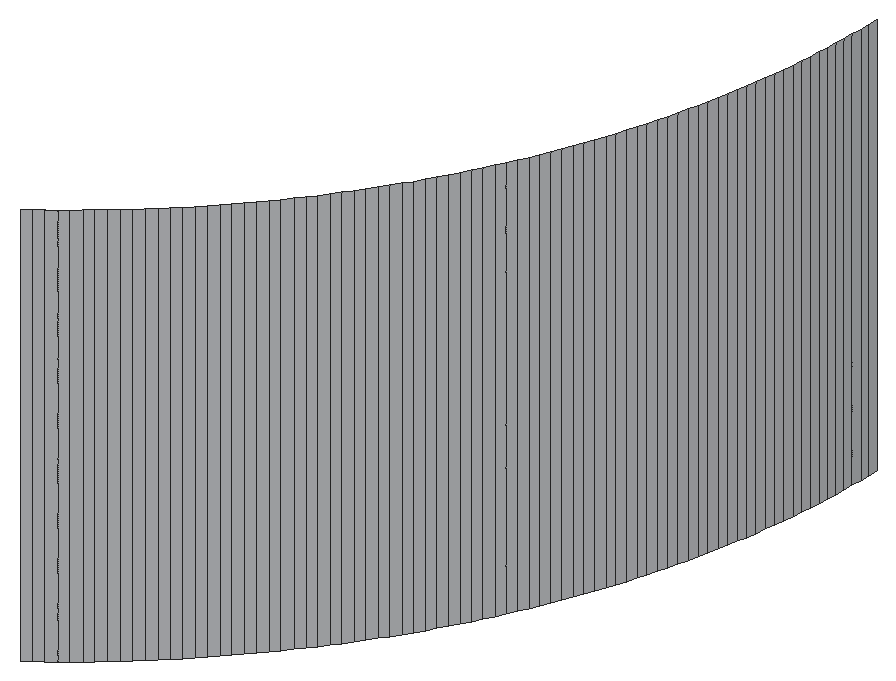
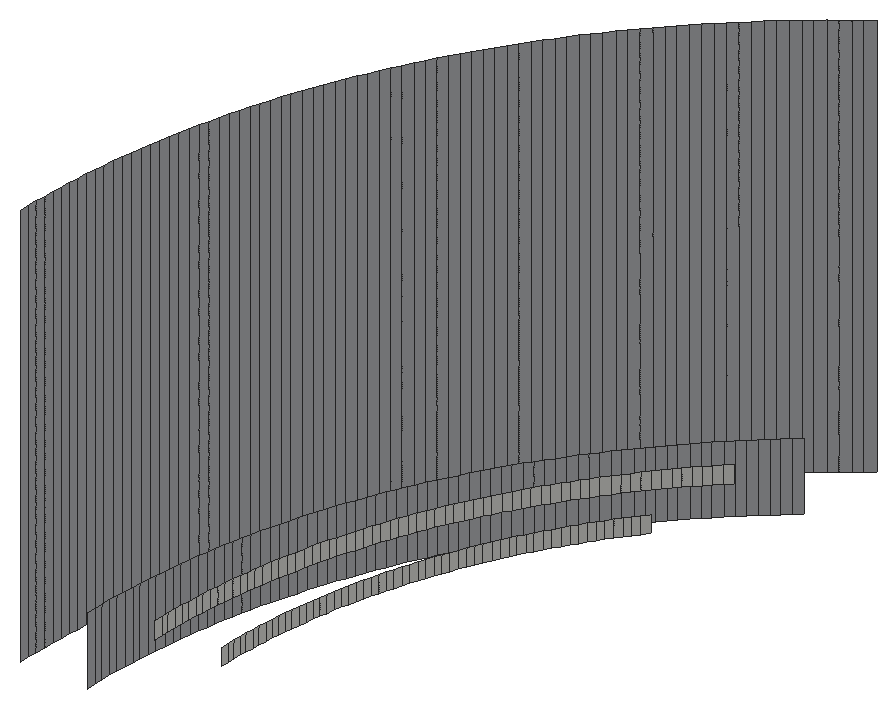
# SketchUp Ruby script. Lengths in inches.
U = 1.inch
M = Sketchup.active_model
def pt(a) = Geom::Point3d.new(a.map { |v| v * U })
def face(e, loops, mat)
  f = e.add_face(loops[0].map { |a| pt(a) })
  loops[1..].each { |l| e.add_face(l.map { |a| pt(a) }).erase! }
  f.material = f.back_material = mat if mat
  f
end
# faces: each face lists its corners as indices into pts; further lists are holes
def faces(e, pts, list, mat = nil) = list.each { |f| face(e, (f[0].is_a?(Array) ? f : [f]).map { |l| l.map { |i| pts[i] } }, mat) }
# xy, xz, yz: faces in a plane at the given z, y or x. An outline is a flat list of corners, or four numbers for a rectangle; further outlines are holes
def ring(l) = l.size == 4 ? [[l[0], l[1]], [l[2], l[1]], [l[2], l[3]], [l[0], l[3]]] : l.each_slice(2).to_a
def flat(e, list, mat, &to3) = list.each { |f| face(e, (f[0].is_a?(Array) ? f : [f]).map { |l| ring(l).map { |u, v| to3.(u, v) } }, mat) }
def xy(e, z, list, mat = nil) = flat(e, list, mat) { |x, y| [x, y, z] }
def xz(e, y, list, mat = nil) = flat(e, list, mat) { |x, z| [x, y, z] }
def yz(e, x, list, mat = nil) = flat(e, list, mat) { |y, z| [x, y, z] }
def lines(e, pts, list) = list.each { |a, b| e.add_line(pt(pts[a]), pt(pts[b])) }
# prism: a flat outline (further loops are holes) pulled along v
def prism(e, loops, v, mat = nil)
  f = face(e, loops, mat); d = Geom::Vector3d.new(v.map { |x| x * U })
  f.pushpull(f.normal.samedirection?(d) ? d.length : -d.length)
end
def box(e, o, s, mat = nil) = prism(e, [[o, [o[0] + s[0], o[1], o[2]], [o[0] + s[0], o[1] + s[1], o[2]], [o[0], o[1] + s[1], o[2]]]], [0, 0, s[2]], mat)
def at(x, y, z, deg = 0) = Geom::Transformation.translation(pt([x, y, z])) * Geom::Transformation.rotation(ORIGIN, Z_AXIS, deg.degrees)
def axes(o, x, y, z) = Geom::Transformation.new([*x, 0, *y, 0, *z, 0, *pt(o).to_a, 1])
def part(name) = M.definitions.add(name)
# library, detail: a bought-in or finely detailed component or shape, given as its bounding box
def library(name, o, s) = part(name).tap { |d| box(d.entities, o, s) }
def detail(e, o, s) = box(e.add_group.entities, o, s)
def put(e, d, t, mat = nil) = e.add_instance(d, t).tap { |i| i.material = mat if mat }
def group(e, t, mat = nil) = e.add_group.tap { |g| g.transformation = t; g.material = mat if mat }.entities
root = M.entities
M.materials.add("1427 AP 686 ARMOUR-N").color = [184, 186, 189]
yz(root,158.99,[[153.27,242,153.49,242.5]])
yz(root,159,[[153.71,242,153.94,242.5]])
yz(root,160.99,[[153.2,242,153.44,242.5]])
yz(root,161,[[153.68,242,153.9375,242.5]])
yz(root,162.99,[[153.13,240,153.39,242]],"1427 AP 686 ARMOUR-N")
yz(root,163,[[153.66,240,153.93,242]],"1427 AP 686 ARMOUR-N")
yz(root,165,[[153.63,240,153.92,252]],"1427 AP 686 ARMOUR-N")
p = [[155.34,134.68,252],[155.11,134.51,252],[155.11,134.51,240],[155.34,134.68,240],[155.57,134.85,252],[155.57,134.85,240],
  [155.8,135.03,252],[155.8,135.03,240],[156.03,135.21,252],[156.03,135.21,240],[156.25,135.4,252],[156.25,135.4,240],
  [156.48,135.58,252],[156.48,135.58,240],[156.7,135.77,252],[156.7,135.77,240],[156.91,135.96,252],[156.91,135.96,240],
  [157.13,136.15,252],[157.13,136.15,240],[157.34,136.35,252],[157.34,136.35,240],[157.55,136.55,252],[157.55,136.55,240],
  [157.76,136.75,252],[157.76,136.75,240],[157.97,136.95,252],[157.97,136.95,240],[158.17,137.16,252],[158.17,137.16,240],
  [155.39,137.28,240],[155.19,137.11,240],[155.19,137.11,242],[155.39,137.28,242],[158.375,137.37,252],[158.375,137.37,240],
  [155.59,137.46,240],[155.59,137.46,242],[158.57,137.58,252],[158.57,137.58,240],[155.79,137.63,240],[155.79,137.63,242],
  [155.98,137.8125,240],[155.98,137.8125,242],[158.77,137.79,252],[158.77,137.79,240],[156.17,138,240],[156.17,138,242],
  [158.96,138.01,252],[158.96,138.01,240],[156.37,138.18,240],[156.37,138.18,242],[159.15,138.23,252],[159.15,138.23,240],
  [156.56,138.37,240],[156.56,138.37,242],[159.34,138.45,252],[159.34,138.45,240],[156.74,138.56,240],[156.74,138.56,242],
  [159.53,138.67,252],[159.53,138.67,240],[156.93,138.75,240],[156.93,138.75,242],[157.11,138.94,240],[157.11,138.94,242],
  [159.71,138.9,252],[159.71,138.9,240],[157.29,139.14,240],[157.29,139.14,242],[159.89,139.125,252],[159.89,139.125,240],
  [157.47,139.34,240],[157.47,139.34,242],[160.07,139.35,252],[160.07,139.35,240],[157.64,139.54,240],[157.64,139.54,242],
  [160.24,139.58,252],[160.24,139.58,240],[157.8125,139.74,240],[157.8125,139.74,242],[160.42,139.82,252],[160.42,139.82,240],
  [157.98,139.94,240],[157.98,139.94,242],[160.58,140.05,252],[160.58,140.05,240],[158.15,140.15,240],[158.15,140.15,242],
  [158.32,140.36,240],[158.32,140.36,242],[160.75,140.29,252],[160.75,140.29,240],[160.91,140.53,252],[160.91,140.53,240],
  [158.48,140.57,240],[158.48,140.57,242],[161.07,140.77,252],[161.07,140.77,240],[158.64,140.78,240],[158.64,140.78,242],
  [158.8,140.99,240],[158.8,140.99,242],[161.23,141.02,252],[161.23,141.02,240],[158.95,141.21,240],[158.95,141.21,242],
  [161.39,141.26,252],[161.39,141.26,240],[159.1,141.43,240],[159.1,141.43,242],[161.54,141.51,252],[161.54,141.51,240],
  [159.25,141.65,240],[159.25,141.65,242],[161.6875,141.76,252],[161.6875,141.76,240],[159.4,141.87,240],[159.4,141.87,242],
  [161.83,142.01,252],[161.83,142.01,240],[159.55,142.09,240],[159.55,142.09,242],[161.97,142.26,252],[161.97,142.26,240],
  [159.6875,142.32,240],[159.6875,142.32,242],[159.83,142.54,240],[159.83,142.54,242],[162.11,142.51,252],[162.11,142.51,240],
  [159.96,142.77,240],[159.96,142.77,242],[162.25,142.77,252],[162.25,142.77,240],[160.1,143,240],[160.1,143,242],
  [162.38,143.03,252],[162.38,143.03,240],[160.23,143.23,240],[160.23,143.23,242],[162.51,143.29,252],[162.51,143.29,240],
  [160.35,143.47,240],[160.35,143.47,242],[162.64,143.55,252],[162.64,143.55,240],[160.48,143.7,240],[160.48,143.7,242],
  [162.76,143.8125,252],[162.76,143.8125,240],[160.6,143.9375,240],[160.6,143.9375,242],[162.88,144.07,252],[162.88,144.07,240],
  [160.72,144.17,240],[160.72,144.17,242],[163,144.34,252],[163,144.34,240],[160.84,144.41,240],[160.84,144.41,242],
  [163.12,144.61,252],[163.12,144.61,240],[160.95,144.65,240],[160.95,144.65,242],[163.23,144.875,252],[163.23,144.875,240],
  [161.0625,144.9,240],[161.0625,144.9,242],[161.17,145.14,240],[161.17,145.14,242],[163.34,145.14,252],[163.34,145.14,240],
  [161.27,145.38,240],[161.27,145.38,242],[163.44,145.41,252],[163.44,145.41,240],[161.375,145.63,240],[161.375,145.63,242],
  [163.54,145.6875,252],[163.54,145.6875,240],[161.47,145.875,240],[161.47,145.875,242],[163.64,145.96,252],[163.64,145.96,240],
  [161.57,146.125,240],[161.57,146.125,242],[163.73,146.23,252],[163.73,146.23,240],[161.66,146.37,240],[161.66,146.37,242],
  [163.82,146.51,252],[163.82,146.51,240],[161.75,146.62,240],[161.75,146.62,242],[163.91,146.78,252],[163.91,146.78,240],
  [161.84,146.875,240],[161.84,146.875,242],[164,147.0625,252],[164,147.0625,240],[161.92,147.125,240],[161.92,147.125,242],
  [162,147.38,240],[162,147.38,242],[164.08,147.34,252],[164.08,147.34,240],[164.16,147.62,252],[164.16,147.62,240],
  [162.08,147.63,240],[162.08,147.63,242],[162.16,147.89,240],[162.16,147.89,242],[164.23,147.9,252],[164.23,147.9,240],
  [162.23,148.14,240],[162.23,148.14,242],[164.3,148.18,252],[164.3,148.18,240],[162.3,148.4,240],[162.3,148.4,242],
  [164.37,148.46,252],[164.37,148.46,240],[162.36,148.66,240],[162.36,148.66,242],[164.43,148.75,252],[164.43,148.75,240],
  [162.42,148.92,240],[162.42,148.92,242],[164.5,149.03,252],[164.5,149.03,240],[162.48,149.18,240],[162.48,149.18,242],
  [164.55,149.3125,252],[164.55,149.3125,240],[162.54,149.4375,240],[162.54,149.4375,242],[164.61,149.6,252],[164.61,149.6,240],
  [162.59,149.7,240],[162.59,149.7,242],[164.66,149.88,252],[164.66,149.88,240],[162.64,149.96,240],[162.64,149.96,242],
  [164.7,150.17,252],[164.7,150.17,240],[162.6875,150.22,240],[162.6875,150.22,242],[162.73,150.48,240],[162.73,150.48,242],
  [164.75,150.46,252],[164.75,150.46,240],[162.77,150.75,240],[162.77,150.75,242],[164.79,150.74,252],[164.79,150.74,240],
  [162.81,151.01,240],[162.81,151.01,242],[164.82,151.03,252],[164.82,151.03,240],[162.84,151.27,240],[162.84,151.27,242],
  [164.86,151.32,252],[164.86,151.32,240],[162.87,151.54,240],[162.87,151.54,242],[164.89,151.61,252],[164.89,151.61,240],
  [162.9,151.8,240],[162.9,151.8,242],[164.91,151.9,252],[164.91,151.9,240],[162.92,152.07,240],[162.92,152.07,242],
  [164.9375,152.1875,252],[164.9375,152.1875,240],[162.94,152.33,240],[162.94,152.33,242],[164.96,152.48,252],[164.96,152.48,240],
  [162.96,152.6,240],[162.96,152.6,242],[164.97,152.76,252],[164.97,152.76,240],[162.97,152.86,240],[162.97,152.86,242],
  [164.98,153.05,252],[164.98,153.05,240],[162.99,153.13,240],[162.99,153.13,242],[164.99,153.34,252],[164.99,153.34,240],
  [165,153.63,252],[165,153.63,240],[163,153.66,240],[162.99,153.39,240],[162.99,153.39,242],[163,153.66,242],
  [155.3125,139.95,242],[155.14,139.78,242],[155.14,139.78,242.5],[155.3125,139.95,242.5],[155.48,140.13,242],[155.48,140.13,242.5],
  [155.64,140.3,242],[155.64,140.3,242.5],[155.81,140.48,242],[155.81,140.48,242.5],[155.97,140.66,242],[155.97,140.66,242.5],
  [156.13,140.84,242],[156.13,140.84,242.5],[156.29,141.03,242],[156.29,141.03,242.5],[156.44,141.21,242],[156.44,141.21,242.5],
  [156.59,141.4,242],[156.59,141.4,242.5],[156.74,141.59,242],[156.74,141.59,242.5],[156.89,141.78,242],[156.89,141.78,242.5],
  [157.04,141.97,242],[157.04,141.97,242.5],[157.18,142.17,242],[157.18,142.17,242.5],[157.32,142.37,242],[157.32,142.37,242.5],
  [157.46,142.5625,242],[157.46,142.5625,242.5],[157.59,142.76,242],[157.59,142.76,242.5],[155.17,142.82,242],[155.3,143,242],
  [155.3,143,242.5],[155.17,142.82,242.5],[157.73,142.96,242],[157.73,142.96,242.5],[155.43,143.17,242],[155.43,143.17,242.5],
  [157.86,143.17,242],[157.86,143.17,242.5],[155.5625,143.34,242],[155.5625,143.34,242.5],[157.99,143.37,242],[157.99,143.37,242.5],
  [155.6875,143.52,242],[155.6875,143.52,242.5],[158.11,143.58,242],[158.11,143.58,242.5],[155.8125,143.7,242],[155.8125,143.7,242.5],
  [158.24,143.79,242],[158.24,143.79,242.5],[155.94,143.88,242],[155.94,143.88,242.5],[158.36,143.99,242],[158.36,143.99,242.5],
  [156.06,144.06,242],[156.06,144.06,242.5],[158.48,144.2,242],[158.48,144.2,242.5],[156.17,144.24,242],[156.17,144.24,242.5],
  [156.29,144.43,242],[156.29,144.43,242.5],[158.59,144.42,242],[158.59,144.42,242.5],[156.4,144.61,242],[156.4,144.61,242.5],
  [158.71,144.63,242],[158.71,144.63,242.5],[156.51,144.8,242],[156.51,144.8,242.5],[158.82,144.84,242],[158.82,144.84,242.5],
  [156.625,144.99,242],[156.625,144.99,242.5],[158.93,145.0625,242],[158.93,145.0625,242.5],[156.73,145.18,242],[156.73,145.18,242.5],
  [159.03,145.28,242],[159.03,145.28,242.5],[156.84,145.37,242],[156.84,145.37,242.5],[159.14,145.5,242],[159.14,145.5,242.5],
  [156.9375,145.56,242],[156.9375,145.56,242.5],[159.24,145.72,242],[159.24,145.72,242.5],[157.04,145.75,242],[157.04,145.75,242.5],
  [159.34,145.9375,242],[159.34,145.9375,242.5],[157.14,145.95,242],[157.14,145.95,242.5],[157.23,146.14,242],[157.23,146.14,242.5],
  [159.43,146.16,242],[159.43,146.16,242.5],[157.32,146.34,242],[157.32,146.34,242.5],[159.52,146.38,242],[159.52,146.38,242.5],
  [157.41,146.54,242],[157.41,146.54,242.5],[159.61,146.61,242],[159.61,146.61,242.5],[157.5,146.74,242],[157.5,146.74,242.5],
  [159.7,146.83,242],[159.7,146.83,242.5],[157.59,146.9375,242],[157.59,146.9375,242.5],[159.78,147.06,242],[159.78,147.06,242.5],
  [157.67,147.14,242],[157.67,147.14,242.5],[157.75,147.34,242],[157.75,147.34,242.5],[159.87,147.29,242],[159.87,147.29,242.5],
  [157.83,147.54,242],[157.83,147.54,242.5],[159.94,147.51,242],[159.94,147.51,242.5],[157.91,147.75,242],[157.91,147.75,242.5],
  [160.02,147.74,242],[160.02,147.74,242.5],[157.98,147.95,242],[157.98,147.95,242.5],[160.09,147.97,242],[160.09,147.97,242.5],
  [158.05,148.16,242],[158.05,148.16,242.5],[160.16,148.21,242],[160.16,148.21,242.5],[158.12,148.36,242],[158.12,148.36,242.5],
  [160.23,148.4375,242],[160.23,148.4375,242.5],[158.18,148.57,242],[158.18,148.57,242.5],[160.3,148.67,242],[160.3,148.67,242.5],
  [158.25,148.78,242],[158.25,148.78,242.5],[160.36,148.9,242],[160.36,148.9,242.5],[158.31,148.99,242],[158.31,148.99,242.5],
  [160.42,149.14,242],[160.42,149.14,242.5],[158.37,149.2,242],[158.37,149.2,242.5],[160.47,149.375,242],[160.47,149.375,242.5],
  [158.42,149.41,242],[158.42,149.41,242.5],[158.48,149.62,242],[158.48,149.62,242.5],[160.53,149.61,242],[160.53,149.61,242.5],
  [158.53,149.83,242],[158.53,149.83,242.5],[160.58,149.85,242],[160.58,149.85,242.5],[158.58,150.04,242],[158.58,150.04,242.5],
  [160.63,150.08,242],[160.63,150.08,242.5],[158.62,150.25,242],[158.62,150.25,242.5],[160.67,150.32,242],[160.67,150.32,242.5],
  [158.66,150.47,242],[158.66,150.47,242.5],[160.71,150.56,242],[160.71,150.56,242.5],[158.7,150.68,242],[158.7,150.68,242.5],
  [160.75,150.8,242],[160.75,150.8,242.5],[158.74,150.89,242],[158.74,150.89,242.5],[160.79,151.03,242],[160.79,151.03,242.5],
  [158.78,151.11,242],[158.78,151.11,242.5],[160.82,151.27,242],[160.82,151.27,242.5],[158.8125,151.32,242],[158.8125,151.32,242.5],
  [158.84,151.54,242],[158.84,151.54,242.5],[160.85,151.51,242],[160.85,151.51,242.5],[158.87,151.76,242],[158.87,151.76,242.5],
  [160.88,151.75,242],[160.88,151.75,242.5],[158.89,151.97,242],[158.89,151.97,242.5],[160.91,151.99,242],[160.91,151.99,242.5],
  [158.92,152.1875,242],[158.92,152.1875,242.5],[160.93,152.24,242],[160.93,152.24,242.5],[158.94,152.4,242],[158.94,152.4,242.5],
  [160.95,152.48,242],[160.95,152.48,242.5],[158.95,152.62,242],[158.95,152.62,242.5],[160.96,152.72,242],[160.96,152.72,242.5],
  [158.97,152.84,242],[158.97,152.84,242.5],[160.98,152.96,242],[160.98,152.96,242.5],[158.98,153.06,242],[158.98,153.06,242.5],
  [160.99,153.2,242],[160.99,153.2,242.5],[158.99,153.27,242],[158.99,153.27,242.5],[161,153.68,242],[160.99,153.44,242],
  [160.99,153.44,242.5],[161,153.68,242.5],[158.99,153.49,242],[159,153.71,242],[159,153.71,242.5],[158.99,153.49,242.5]]
faces(root,p,[[0,1,2,3],[4,0,3,5],[6,4,5,7],[8,6,7,9],[10,8,9,11],[12,10,11,13],[14,12,13,15],[16,14,15,17],
  [18,16,17,19],[20,18,19,21],[22,20,21,23],[24,22,23,25],[26,24,25,27],[28,26,27,29],[30,31,32,33],[34,28,29,35],
  [36,30,33,37],[38,34,35,39],[40,36,37,41],[42,40,41,43],[44,38,39,45],[46,42,43,47],[48,44,45,49],[50,46,47,51],
  [52,48,49,53],[54,50,51,55],[56,52,53,57],[58,54,55,59],[60,56,57,61],[62,58,59,63],[64,62,63,65],[66,60,61,67],
  [68,64,65,69],[70,66,67,71],[72,68,69,73],[74,70,71,75],[76,72,73,77],[78,74,75,79],[80,76,77,81],[82,78,79,83],
  [84,80,81,85],[86,82,83,87],[88,84,85,89],[90,88,89,91],[92,86,87,93],[94,92,93,95],[96,90,91,97],[98,94,95,99],
  [100,96,97,101],[102,100,101,103],[104,98,99,105],[106,102,103,107],[108,104,105,109],[110,106,107,111],[112,108,109,113],[114,110,111,115],
  [116,112,113,117],[118,114,115,119],[120,116,117,121],[122,118,119,123],[124,120,121,125],[126,122,123,127],[128,126,127,129],[130,124,125,131],
  [132,128,129,133],[134,130,131,135],[136,132,133,137],[138,134,135,139],[140,136,137,141],[142,138,139,143],[144,140,141,145],[146,142,143,147],
  [148,144,145,149],[150,146,147,151],[152,148,149,153],[154,150,151,155],[156,152,153,157],[158,154,155,159],[160,156,157,161],[162,158,159,163],
  [164,160,161,165],[166,162,163,167],[168,164,165,169],[170,168,169,171],[172,166,167,173],[174,170,171,175],[176,172,173,177],[178,174,175,179],
  [180,176,177,181],[182,178,179,183],[184,180,181,185],[186,182,183,187],[188,184,185,189],[190,186,187,191],[192,188,189,193],[194,190,191,195],
  [196,192,193,197],[198,194,195,199],[200,196,197,201],[202,198,199,203],[204,202,203,205],[206,200,201,207],[208,206,207,209],[210,204,205,211],
  [212,210,211,213],[214,208,209,215],[216,212,213,217],[218,214,215,219],[220,216,217,221],[222,218,219,223],[224,220,221,225],[226,222,223,227],
  [228,224,225,229],[230,226,227,231],[232,228,229,233],[234,230,231,235],[236,232,233,237],[238,234,235,239],[240,236,237,241],[242,238,239,243],
  [244,240,241,245],[246,242,243,247],[248,244,245,249],[250,248,249,251],[252,246,247,253],[254,250,251,255],[256,252,253,257],[258,254,255,259],
  [260,256,257,261],[262,258,259,263],[264,260,261,265],[266,262,263,267],[268,264,265,269],[270,266,267,271],[272,268,269,273],[274,270,271,275],
  [276,272,273,277],[278,274,275,279],[280,276,277,281],[282,278,279,283],[284,280,281,285],[286,282,283,287],[288,284,285,289],[290,286,287,291],
  [292,288,289,293],[294,292,293,295],[296,297,298,299]],"1427 AP 686 ARMOUR-N")
faces(root,p,[[300,301,302,303],[304,300,303,305],[306,304,305,307],[308,306,307,309],[310,308,309,311],[312,310,311,313],[314,312,313,315],[316,314,315,317],
  [318,316,317,319],[320,318,319,321],[322,320,321,323],[324,322,323,325],[326,324,325,327],[328,326,327,329],[330,328,329,331],[332,330,331,333],
  [334,335,336,337],[338,332,333,339],[335,340,341,336],[342,338,339,343],[340,344,345,341],[346,342,343,347],[344,348,349,345],[350,346,347,351],
  [348,352,353,349],[354,350,351,355],[352,356,357,353],[358,354,355,359],[356,360,361,357],[362,358,359,363],[360,364,365,361],[364,366,367,365],
  [368,362,363,369],[366,370,371,367],[372,368,369,373],[370,374,375,371],[376,372,373,377],[374,378,379,375],[380,376,377,381],[378,382,383,379],
  [384,380,381,385],[382,386,387,383],[388,384,385,389],[386,390,391,387],[392,388,389,393],[390,394,395,391],[396,392,393,397],[394,398,399,395],
  [398,400,401,399],[402,396,397,403],[400,404,405,401],[406,402,403,407],[404,408,409,405],[410,406,407,411],[408,412,413,409],[414,410,411,415],
  [412,416,417,413],[418,414,415,419],[416,420,421,417],[420,422,423,421],[424,418,419,425],[422,426,427,423],[428,424,425,429],[426,430,431,427],
  [432,428,429,433],[430,434,435,431],[436,432,433,437],[434,438,439,435],[440,436,437,441],[438,442,443,439],[444,440,441,445],[442,446,447,443],
  [448,444,445,449],[446,450,451,447],[452,448,449,453],[450,454,455,451],[456,452,453,457],[454,458,459,455],[460,456,457,461],[458,462,463,459],
  [462,464,465,463],[466,460,461,467],[464,468,469,465],[470,466,467,471],[468,472,473,469],[474,470,471,475],[472,476,477,473],[478,474,475,479],
  [476,480,481,477],[482,478,479,483],[480,484,485,481],[486,482,483,487],[484,488,489,485],[490,486,487,491],[488,492,493,489],[494,490,491,495],
  [492,496,497,493],[496,498,499,497],[500,494,495,501],[498,502,503,499],[504,500,501,505],[502,506,507,503],[508,504,505,509],[506,510,511,507],
  [512,508,509,513],[510,514,515,511],[516,512,513,517],[514,518,519,515],[520,516,517,521],[518,522,523,519],[524,520,521,525],[522,526,527,523],
  [528,524,525,529],[526,530,531,527],[532,533,534,535],[536,537,538,539]])
